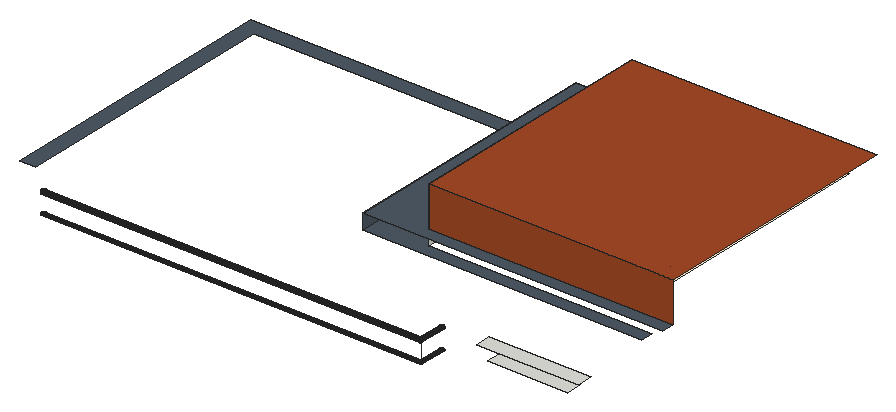
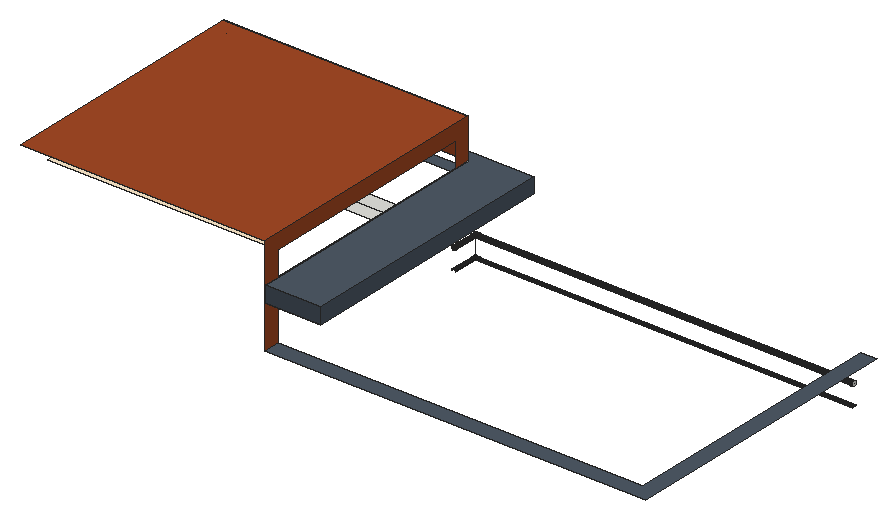
# SketchUp Ruby script. Lengths in inches.
U = 1.inch
M = Sketchup.active_model
def pt(a) = Geom::Point3d.new(a.map { |v| v * U })
def face(e, loops, mat)
  f = e.add_face(loops[0].map { |a| pt(a) })
  loops[1..].each { |l| e.add_face(l.map { |a| pt(a) }).erase! }
  f.material = f.back_material = mat if mat
  f
end
# faces: each face lists its corners as indices into pts; further lists are holes
def faces(e, pts, list, mat = nil) = list.each { |f| face(e, (f[0].is_a?(Array) ? f : [f]).map { |l| l.map { |i| pts[i] } }, mat) }
# xy, xz, yz: faces in a plane at the given z, y or x. An outline is a flat list of corners, or four numbers for a rectangle; further outlines are holes
def ring(l) = l.size == 4 ? [[l[0], l[1]], [l[2], l[1]], [l[2], l[3]], [l[0], l[3]]] : l.each_slice(2).to_a
def flat(e, list, mat, &to3) = list.each { |f| face(e, (f[0].is_a?(Array) ? f : [f]).map { |l| ring(l).map { |u, v| to3.(u, v) } }, mat) }
def xy(e, z, list, mat = nil) = flat(e, list, mat) { |x, y| [x, y, z] }
def xz(e, y, list, mat = nil) = flat(e, list, mat) { |x, z| [x, y, z] }
def yz(e, x, list, mat = nil) = flat(e, list, mat) { |y, z| [x, y, z] }
def lines(e, pts, list) = list.each { |a, b| e.add_line(pt(pts[a]), pt(pts[b])) }
# prism: a flat outline (further loops are holes) pulled along v
def prism(e, loops, v, mat = nil)
  f = face(e, loops, mat); d = Geom::Vector3d.new(v.map { |x| x * U })
  f.pushpull(f.normal.samedirection?(d) ? d.length : -d.length)
end
def box(e, o, s, mat = nil) = prism(e, [[o, [o[0] + s[0], o[1], o[2]], [o[0] + s[0], o[1] + s[1], o[2]], [o[0], o[1] + s[1], o[2]]]], [0, 0, s[2]], mat)
def at(x, y, z, deg = 0) = Geom::Transformation.translation(pt([x, y, z])) * Geom::Transformation.rotation(ORIGIN, Z_AXIS, deg.degrees)
def axes(o, x, y, z) = Geom::Transformation.new([*x, 0, *y, 0, *z, 0, *pt(o).to_a, 1])
def part(name) = M.definitions.add(name)
# library, detail: a bought-in or finely detailed component or shape, given as its bounding box
def library(name, o, s) = part(name).tap { |d| box(d.entities, o, s) }
def detail(e, o, s) = box(e.add_group.entities, o, s)
def put(e, d, t, mat = nil) = e.add_instance(d, t).tap { |i| i.material = mat if mat }
def group(e, t, mat = nil) = e.add_group.tap { |g| g.transformation = t; g.material = mat if mat }.entities
root = M.entities
M.materials.add("[0029_BlanchedAlmond]").color = [255, 235, 205]
M.materials.add("[0047_Khaki]").color = [240, 230, 140]
M.materials.add("[0111_SlateGray]").color = [79, 90, 102]
M.materials.add("[0136_Charcoal]").color = [35, 35, 35]
M.materials.add("[Cladding Siding Tan]").color = [162, 73, 37]
xy(root,2520,[[2669.375,1132.62,2981.375,1192.62]])
xy(root,2536.5,[[2448.125,1082.62,2448.96,1082.66,2449.79,1082.79,2450.6,1083.01,2451.38,1083.31,2452.125,1083.6875,2452.83,1084.15,2453.48,1084.67,2454.07,1085.26,2454.6,1085.92,2455.05,1086.62,2455.43,1087.36,2455.73,1088.15,2455.95,1088.95,2456.08,1089.78,2456.125,1090.62,2456.08,1091.45,2455.95,1092.28,2455.73,1093.09,2455.43,1093.87,2455.05,1094.62,2454.6,1095.32,2454.07,1095.97,2453.48,1096.5625,2452.83,1097.09,2452.125,1097.55,2451.38,1097.93,2450.6,1098.23,2449.79,1098.44,2448.96,1098.57,2448.125,1098.62,2447.29,1098.57,2446.46,1098.44,2445.65,1098.23,2444.87,1097.93,2444.125,1097.55,2443.42,1097.09,2442.77,1096.5625,2442.18,1095.97,2441.65,1095.32,2441.19,1094.62,2440.81,1093.87,2440.51,1093.09,2440.3,1092.28,2440.17,1091.45,2440.125,1090.62,2440.17,1089.78,2440.3,1088.95,2440.51,1088.15,2440.81,1087.36,2441.19,1086.62,2441.65,1085.92,2442.18,1085.26,2442.77,1084.67,2443.42,1084.15,2444.125,1083.6875,2444.87,1083.31,2445.65,1083.01,2446.46,1082.79,2447.29,1082.66]])
xy(root,2562,[[2627.375,1132.62,3023.375,1192.62]])
xy(root,2630.25,[[917.375,1060.62,977.375,1060.62,977.375,2116.62,2393.375,2116.62,2393.375,2176.62,917.375,2176.62]],"[0111_SlateGray]")
xy(root,2796,[[2275.57,1241.83,2272.48,1242.38,2269.65,1243.71,2267.25,1245.73,2265.46,1248.3,2264.4,1251.25,2264.13,1254.37,2264.68,1257.46,2266.01,1260.29,2268.03,1262.6875,2270.6,1264.48,2273.55,1265.54,2276.67,1265.81,2279.75,1265.26,2282.59,1263.93,2284.98,1261.91,2286.77,1259.34,2287.84,1256.39,2288.11,1253.27,2287.55,1250.19,2286.22,1247.35,2284.2,1244.95,2281.63,1243.16,2278.6875,1242.1],[2275.57,1421.83,2272.48,1422.38,2269.65,1423.71,2267.25,1425.73,2265.46,1428.3,2264.4,1431.25,2264.13,1434.37,2264.68,1437.46,2266.01,1440.29,2268.03,1442.6875,2270.6,1444.48,2273.55,1445.54,2276.67,1445.81,2279.75,1445.26,2282.59,1443.93,2284.98,1441.91,2286.77,1439.34,2287.84,1436.39,2288.11,1433.27,2287.55,1430.19,2286.22,1427.35,2284.2,1424.95,2281.63,1423.16,2278.6875,1422.1],[2275.57,1601.83,2272.48,1602.38,2269.65,1603.71,2267.25,1605.73,2265.46,1608.3,2264.4,1611.25,2264.13,1614.37,2264.68,1617.46,2266.01,1620.29,2268.03,1622.6875,2270.6,1624.48,2273.55,1625.54,2276.67,1625.81,2279.75,1625.26,2282.59,1623.93,2284.98,1621.91,2286.77,1619.34,2287.84,1616.39,2288.11,1613.27,2287.55,1610.19,2286.22,1607.35,2284.2,1604.95,2281.63,1603.16,2278.6875,1602.1],[2275.57,1781.83,2272.48,1782.38,2269.65,1783.71,2267.25,1785.73,2265.46,1788.3,2264.4,1791.25,2264.13,1794.37,2264.68,1797.46,2266.01,1800.29,2268.03,1802.6875,2270.6,1804.48,2273.55,1805.54,2276.67,1805.81,2279.75,1805.26,2282.59,1803.93,2284.98,1801.91,2286.77,1799.34,2287.84,1796.39,2288.11,1793.27,2287.55,1790.19,2286.22,1787.35,2284.2,1784.95,2281.63,1783.16,2278.6875,1782.1],[2275.57,1961.83,2272.48,1962.38,2269.65,1963.71,2267.25,1965.73,2265.46,1968.3,2264.4,1971.25,2264.13,1974.37,2264.68,1977.46,2266.01,1980.29,2268.03,1982.6875,2270.6,1984.48,2273.55,1985.54,2276.67,1985.81,2279.75,1985.26,2282.59,1983.93,2284.98,1981.91,2286.77,1979.34,2287.84,1976.39,2288.11,1973.27,2287.55,1970.19,2286.22,1967.35,2284.2,1964.95,2281.63,1963.16,2278.6875,1962.1]],"[0047_Khaki]")
xy(root,2796,[[[2177.375,1144.62,2177.375,2176.62,2393.375,2176.62,2393.375,1192.62,3257.375,1192.62,3257.375,1144.62],[2275.57,1421.83,2278.6875,1422.1,2281.63,1423.16,2284.2,1424.95,2286.22,1427.35,2287.55,1430.19,2288.11,1433.27,2287.84,1436.39,2286.77,1439.34,2284.98,1441.91,2282.59,1443.93,2279.75,1445.26,2276.67,1445.81,2273.55,1445.54,2270.6,1444.48,2268.03,1442.6875,2266.01,1440.29,2264.68,1437.46,2264.13,1434.37,2264.4,1431.25,2265.46,1428.3,2267.25,1425.73,2269.65,1423.71,2272.48,1422.38],[2275.57,1781.83,2278.6875,1782.1,2281.63,1783.16,2284.2,1784.95,2286.22,1787.35,2287.55,1790.19,2288.11,1793.27,2287.84,1796.39,2286.77,1799.34,2284.98,1801.91,2282.59,1803.93,2279.75,1805.26,2276.67,1805.81,2273.55,1805.54,2270.6,1804.48,2268.03,1802.6875,2266.01,1800.29,2264.68,1797.46,2264.13,1794.37,2264.4,1791.25,2265.46,1788.3,2267.25,1785.73,2269.65,1783.71,2272.48,1782.38],[2275.57,1601.83,2278.6875,1602.1,2281.63,1603.16,2284.2,1604.95,2286.22,1607.35,2287.55,1610.19,2288.11,1613.27,2287.84,1616.39,2286.77,1619.34,2284.98,1621.91,2282.59,1623.93,2279.75,1625.26,2276.67,1625.81,2273.55,1625.54,2270.6,1624.48,2268.03,1622.6875,2266.01,1620.29,2264.68,1617.46,2264.13,1614.37,2264.4,1611.25,2265.46,1608.3,2267.25,1605.73,2269.65,1603.71,2272.48,1602.38],[2275.57,1961.83,2278.6875,1962.1,2281.63,1963.16,2284.2,1964.95,2286.22,1967.35,2287.55,1970.19,2288.11,1973.27,2287.84,1976.39,2286.77,1979.34,2284.98,1981.91,2282.59,1983.93,2279.75,1985.26,2276.67,1985.81,2273.55,1985.54,2270.6,1984.48,2268.03,1982.6875,2266.01,1980.29,2264.68,1977.46,2264.13,1974.37,2264.4,1971.25,2265.46,1968.3,2267.25,1965.73,2269.65,1963.71,2272.48,1962.38],[2275.57,1241.83,2278.6875,1242.1,2281.63,1243.16,2284.2,1244.95,2286.22,1247.35,2287.55,1250.19,2288.11,1253.27,2287.84,1256.39,2286.77,1259.34,2284.98,1261.91,2282.59,1263.93,2279.75,1265.26,2276.67,1265.81,2273.55,1265.54,2270.6,1264.48,2268.03,1262.6875,2266.01,1260.29,2264.68,1257.46,2264.13,1254.37,2264.4,1251.25,2265.46,1248.3,2267.25,1245.73,2269.65,1243.71,2272.48,1242.38]]],"[0111_SlateGray]")
xy(root,2856,[[2177.375,1144.62,3341.375,1144.62,3341.375,1192.62,2393.375,1192.62,2393.375,2176.62,2177.375,2176.62]],"[0111_SlateGray]")
xy(root,2952,[[2393.375,1252.62,3281.375,2116.62]],"[0029_BlanchedAlmond]")
xy(root,3012,[[2393.375,1192.62,3341.375,2176.62]],"[Cladding Siding Tan]")
xz(root,1192.62,[[2393.375,2856,3341.375,3012]],"[Cladding Siding Tan]")
xz(root,2176.62,[[2177.375,2796,2393.375,2856]],"[0111_SlateGray]")
yz(root,977.375,[[1090.62,2527,1089.78,2527.04,1088.95,2527.17,1088.15,2527.39,1087.36,2527.69,1086.62,2528.07,1085.92,2528.53,1085.26,2529.05,1084.67,2529.65,1084.15,2530.3,1083.6875,2531,1083.31,2531.75,1083.01,2532.53,1082.79,2533.34,1082.66,2534.16,1082.62,2535,1082.66,2535.84,1082.79,2536.66,1083.01,2537.47,1083.31,2538.25,1083.6875,2539,1084.15,2539.7,1084.67,2540.35,1085.26,2540.95,1085.92,2541.47,1086.62,2541.93,1087.36,2542.31,1088.15,2542.61,1088.95,2542.83,1089.78,2542.96,1090.62,2543,1091.45,2542.96,1092.28,2542.83,1093.09,2542.61,1093.87,2542.31,1094.62,2541.93,1095.32,2541.47,1095.97,2540.95,1096.5625,2540.35,1097.09,2539.7,1097.55,2539,1097.93,2538.25,1098.23,2537.47,1098.44,2536.66,1098.57,2535.84,1098.62,2535,1098.57,2534.16,1098.44,2533.34,1098.23,2532.53,1097.93,2531.75,1097.55,2531,1097.09,2530.3,1096.5625,2529.65,1095.97,2529.05,1095.32,2528.53,1094.62,2528.07,1093.87,2527.69,1093.09,2527.39,1092.28,2527.17,1091.45,2527.04]])
yz(root,2177.375,[[1144.62,2796,2176.62,2856]],"[0111_SlateGray]")
yz(root,2393.375,[[1192.62,2796,1252.62,2856],[1252.62,2796,2116.62,2856],[2116.62,2796,2176.62,2856]])
yz(root,2393.375,[[2116.62,2630.25,2176.62,2796],[1192.62,2856,1192.62,3012,2176.62,3012,2176.62,2856,2116.62,2856,2116.62,2952,1252.62,2952,1252.62,2856]],"[Cladding Siding Tan]")
p = [[977.375,1083.01,2456.47],[977.375,1082.79,2455.66],[2446.46,1082.79,2455.66],[2449.79,1082.79,2455.66],[2455.95,1082.79,2455.66],[2455.73,1083.01,2456.47],
  [2450.6,1083.01,2456.47],[2445.65,1083.01,2456.47],[2455.95,1088.95,2455.66],[2455.95,1092.28,2455.66],[2455.95,1192.62,2455.66],[2455.73,1192.62,2456.47],
  [2455.73,1093.09,2456.47],[2455.73,1088.15,2456.47],[977.375,1098.44,2455.66],[977.375,1098.23,2456.47],[2440.51,1098.23,2456.47],[2440.3,1098.44,2455.66],
  [2440.51,1192.62,2456.47],[2440.3,1192.62,2455.66],[977.375,1083.31,2457.25],[2455.43,1083.31,2457.25],[2451.38,1083.31,2457.25],[2444.87,1083.31,2457.25],
  [2455.43,1192.62,2457.25],[2455.43,1093.87,2457.25],[2455.43,1087.36,2457.25],[977.375,1097.93,2457.25],[2440.81,1097.93,2457.25],[2440.81,1192.62,2457.25],
  [977.375,1083.6875,2458],[2455.05,1083.6875,2458],[2452.125,1083.6875,2458],[2444.125,1083.6875,2458],[2455.05,1192.62,2458],[2455.05,1094.62,2458],
  [2455.05,1086.62,2458],[977.375,1097.55,2458],[2441.19,1097.55,2458],[2441.19,1192.62,2458],[977.375,1084.15,2458.7],[2454.6,1084.15,2458.7],
  [2452.83,1084.15,2458.7],[2443.42,1084.15,2458.7],[2454.6,1192.62,2458.7],[2454.6,1095.32,2458.7],[2454.6,1085.92,2458.7],[977.375,1097.09,2458.7],
  [2441.65,1097.09,2458.7],[2441.65,1192.62,2458.7],[977.375,1084.67,2459.35],[2454.07,1084.67,2459.35],[2453.48,1084.67,2459.35],[2442.77,1084.67,2459.35],
  [2454.07,1192.62,2459.35],[2454.07,1095.97,2459.35],[2454.07,1085.26,2459.35],[977.375,1096.5625,2459.35],[2442.18,1096.5625,2459.35],[2442.18,1192.62,2459.35],
  [977.375,1085.26,2459.95],[2453.48,1085.26,2459.95],[2442.18,1085.26,2459.95],[2453.48,1192.62,2459.95],[2453.48,1096.5625,2459.95],[977.375,1095.97,2459.95],
  [2442.18,1095.97,2459.95],[2442.77,1095.97,2459.95],[2442.77,1096.5625,2459.95],[2442.77,1192.62,2459.95],[977.375,1085.92,2460.47],[2452.83,1085.92,2460.47],
  [2441.65,1085.92,2460.47],[2452.83,1192.62,2460.47],[2452.83,1097.09,2460.47],[977.375,1095.32,2460.47],[2441.65,1095.32,2460.47],[2443.42,1095.32,2460.47],
  [2443.42,1097.09,2460.47],[2443.42,1192.62,2460.47],[977.375,1086.62,2460.93],[2452.125,1086.62,2460.93],[2441.19,1086.62,2460.93],[2452.125,1192.62,2460.93],
  [2452.125,1097.55,2460.93],[977.375,1094.62,2460.93],[2441.19,1094.62,2460.93],[2444.125,1094.62,2460.93],[2444.125,1097.55,2460.93],[2444.125,1192.62,2460.93],
  [977.375,1087.36,2461.31],[2451.38,1087.36,2461.31],[2440.81,1087.36,2461.31],[2451.38,1192.62,2461.31],[2451.38,1097.93,2461.31],[977.375,1093.87,2461.31],
  [2440.81,1093.87,2461.31],[2444.87,1093.87,2461.31],[2444.87,1097.93,2461.31],[2444.87,1192.62,2461.31],[977.375,1088.15,2461.61],[2450.6,1088.15,2461.61],
  [2440.51,1088.15,2461.61],[2450.6,1192.62,2461.61],[2450.6,1098.23,2461.61],[977.375,1093.09,2461.61],[2440.51,1093.09,2461.61],[2445.65,1093.09,2461.61],
  [2445.65,1098.23,2461.61],[2445.65,1192.62,2461.61],[977.375,1088.95,2461.83],[2449.79,1088.95,2461.83],[2440.3,1088.95,2461.83],[2449.79,1192.62,2461.83],
  [2449.79,1098.44,2461.83],[977.375,1092.28,2461.83],[2440.3,1092.28,2461.83],[2446.46,1092.28,2461.83],[2446.46,1098.44,2461.83],[2446.46,1192.62,2461.83],
  [977.375,1089.78,2461.96],[2448.96,1089.78,2461.96],[2440.17,1089.78,2461.96],[2448.96,1192.62,2461.96],[2448.96,1098.57,2461.96],[977.375,1091.45,2461.96],
  [2440.17,1091.45,2461.96],[2447.29,1091.45,2461.96],[2447.29,1098.57,2461.96],[2447.29,1192.62,2461.96],[977.375,1090.62,2462],[2448.125,1090.62,2462],
  [2440.125,1090.62,2462],[2448.125,1192.62,2462],[2448.125,1098.62,2462],[977.375,1088.95,2527.17],[977.375,1089.78,2527.04],[2440.17,1089.78,2527.04],
  [2448.96,1089.78,2527.04],[2449.79,1088.95,2527.17],[2440.3,1088.95,2527.17],[2448.96,1098.57,2527.04],[2448.96,1192.62,2527.04],[2449.79,1192.62,2527.17],
  [2449.79,1098.44,2527.17],[977.375,1090.62,2527],[2440.125,1090.62,2527],[2448.125,1090.62,2527],[2448.125,1098.62,2527],[2448.125,1192.62,2527],
  [977.375,1091.45,2527.04],[2440.17,1091.45,2527.04],[2447.29,1091.45,2527.04],[2447.29,1098.57,2527.04],[2447.29,1192.62,2527.04],[977.375,1092.28,2527.17],
  [2440.3,1092.28,2527.17],[2446.46,1092.28,2527.17],[2446.46,1098.44,2527.17],[2446.46,1192.62,2527.17],[977.375,1088.15,2527.39],[2450.6,1088.15,2527.39],
  [2440.51,1088.15,2527.39],[2450.6,1192.62,2527.39],[2450.6,1098.23,2527.39],[977.375,1093.09,2527.39],[2440.51,1093.09,2527.39],[2445.65,1093.09,2527.39],
  [2445.65,1098.23,2527.39],[2445.65,1192.62,2527.39],[977.375,1087.36,2527.69],[2451.38,1087.36,2527.69],[2440.81,1087.36,2527.69],[2451.38,1192.62,2527.69],
  [2451.38,1097.93,2527.69],[977.375,1093.87,2527.69],[2440.81,1093.87,2527.69],[2444.87,1093.87,2527.69],[2444.87,1097.93,2527.69],[2444.87,1192.62,2527.69],
  [977.375,1086.62,2528.07],[2452.125,1086.62,2528.07],[2441.19,1086.62,2528.07],[2452.125,1192.62,2528.07],[2452.125,1097.55,2528.07],[977.375,1094.62,2528.07],
  [2441.19,1094.62,2528.07],[2444.125,1094.62,2528.07],[2444.125,1097.55,2528.07],[2444.125,1192.62,2528.07],[977.375,1085.92,2528.53],[2452.83,1085.92,2528.53],
  [2441.65,1085.92,2528.53],[2452.83,1192.62,2528.53],[2452.83,1097.09,2528.53],[977.375,1095.32,2528.53],[2441.65,1095.32,2528.53],[2443.42,1095.32,2528.53],
  [2443.42,1097.09,2528.53],[2443.42,1192.62,2528.53],[977.375,1085.26,2529.05],[2453.48,1085.26,2529.05],[2442.18,1085.26,2529.05],[2453.48,1192.62,2529.05],
  [2453.48,1096.5625,2529.05],[977.375,1095.97,2529.05],[2442.18,1095.97,2529.05],[2442.77,1095.97,2529.05],[2442.77,1096.5625,2529.05],[2442.77,1192.62,2529.05],
  [977.375,1084.67,2529.65],[2454.07,1084.67,2529.65],[2453.48,1084.67,2529.65],[2442.77,1084.67,2529.65],[2454.07,1192.62,2529.65],[2454.07,1095.97,2529.65],
  [2454.07,1085.26,2529.65],[977.375,1096.5625,2529.65],[2442.18,1096.5625,2529.65],[2442.18,1192.62,2529.65],[977.375,1084.15,2530.3],[2454.6,1084.15,2530.3],
  [2452.83,1084.15,2530.3],[2443.42,1084.15,2530.3],[2454.6,1192.62,2530.3],[2454.6,1095.32,2530.3],[2454.6,1085.92,2530.3],[977.375,1097.09,2530.3],
  [2441.65,1097.09,2530.3],[2441.65,1192.62,2530.3],[977.375,1083.6875,2531],[2455.05,1083.6875,2531],[2452.125,1083.6875,2531],[2444.125,1083.6875,2531],
  [2455.05,1192.62,2531],[2455.05,1094.62,2531],[2455.05,1086.62,2531],[977.375,1097.55,2531],[2441.19,1097.55,2531],[2441.19,1192.62,2531],
  [977.375,1083.31,2531.75],[2455.43,1083.31,2531.75],[2451.38,1083.31,2531.75],[2444.87,1083.31,2531.75],[2455.43,1192.62,2531.75],[2455.43,1093.87,2531.75],
  [2455.43,1087.36,2531.75],[977.375,1097.93,2531.75],[2440.81,1097.93,2531.75],[2440.81,1192.62,2531.75],[977.375,1083.01,2532.53],[2455.73,1083.01,2532.53],
  [2450.6,1083.01,2532.53],[2445.65,1083.01,2532.53],[2455.73,1192.62,2532.53],[2455.73,1093.09,2532.53],[2455.73,1088.15,2532.53],[977.375,1098.23,2532.53],
  [2440.51,1098.23,2532.53],[2440.51,1192.62,2532.53],[977.375,1082.79,2533.34],[2455.95,1082.79,2533.34],[2449.79,1082.79,2533.34],[2446.46,1082.79,2533.34],
  [2455.95,1192.62,2533.34],[2455.95,1092.28,2533.34],[2455.95,1088.95,2533.34],[977.375,1098.44,2533.34],[2440.3,1098.44,2533.34],[2440.3,1192.62,2533.34],
  [977.375,1082.66,2534.16],[2456.08,1082.66,2534.16],[2448.96,1082.66,2534.16],[2447.29,1082.66,2534.16],[2456.08,1192.62,2534.16],[2456.08,1091.45,2534.16],
  [2456.08,1089.78,2534.16],[977.375,1098.57,2534.16],[2440.17,1098.57,2534.16],[2440.17,1192.62,2534.16],[977.375,1082.62,2535],[2456.125,1082.62,2535],
  [2448.125,1082.62,2535],[2456.125,1192.62,2535],[2456.125,1090.62,2535],[977.375,1098.62,2535],[2440.125,1098.62,2535],[2440.125,1192.62,2535],
  [977.375,1082.66,2535.84],[2456.08,1082.66,2535.84],[2448.96,1082.66,2535.84],[2447.29,1082.66,2535.84],[2456.08,1192.62,2535.84],[2456.08,1091.45,2535.84],
  [2456.08,1089.78,2535.84],[977.375,1098.57,2535.84],[2440.17,1098.57,2535.84],[2440.17,1192.62,2535.84],[977.375,1082.79,2536.66],[2455.95,1082.79,2536.66],
  [2449.79,1082.79,2536.66],[2446.46,1082.79,2536.66],[2455.95,1192.62,2536.66],[2455.95,1092.28,2536.66],[2455.95,1088.95,2536.66],[977.375,1098.44,2536.66],
  [2440.3,1098.44,2536.66],[2440.3,1192.62,2536.66],[977.375,1083.01,2537.47],[2455.73,1083.01,2537.47],[2450.6,1083.01,2537.47],[2445.65,1083.01,2537.47],
  [2455.73,1192.62,2537.47],[2455.73,1093.09,2537.47],[2455.73,1088.15,2537.47],[977.375,1098.23,2537.47],[2440.51,1098.23,2537.47],[2440.51,1192.62,2537.47],
  [977.375,1083.31,2538.25],[2455.43,1083.31,2538.25],[2451.38,1083.31,2538.25],[2444.87,1083.31,2538.25],[2455.43,1192.62,2538.25],[2455.43,1093.87,2538.25],
  [2455.43,1087.36,2538.25],[977.375,1097.93,2538.25],[2440.81,1097.93,2538.25],[2440.81,1192.62,2538.25],[977.375,1083.6875,2539],[2455.05,1083.6875,2539],
  [2452.125,1083.6875,2539],[2444.125,1083.6875,2539],[2455.05,1192.62,2539],[2455.05,1094.62,2539],[2455.05,1086.62,2539],[977.375,1097.55,2539],
  [2441.19,1097.55,2539],[2441.19,1192.62,2539],[977.375,1084.15,2539.7],[2454.6,1084.15,2539.7],[2452.83,1084.15,2539.7],[2443.42,1084.15,2539.7],
  [2454.6,1192.62,2539.7],[2454.6,1095.32,2539.7],[2454.6,1085.92,2539.7],[977.375,1097.09,2539.7],[2441.65,1097.09,2539.7],[2441.65,1192.62,2539.7],
  [977.375,1084.67,2540.35],[2454.07,1084.67,2540.35],[2453.48,1084.67,2540.35],[2442.77,1084.67,2540.35],[2454.07,1192.62,2540.35],[2454.07,1095.97,2540.35],
  [2454.07,1085.26,2540.35],[977.375,1096.5625,2540.35],[2442.18,1096.5625,2540.35],[2442.18,1192.62,2540.35],[977.375,1085.26,2540.95],[2453.48,1085.26,2540.95],
  [2442.18,1085.26,2540.95],[2453.48,1192.62,2540.95],[2453.48,1096.5625,2540.95],[977.375,1095.97,2540.95],[2442.18,1095.97,2540.95],[2442.77,1095.97,2540.95],
  [2442.77,1096.5625,2540.95],[2442.77,1192.62,2540.95],[977.375,1085.92,2541.47],[2452.83,1085.92,2541.47],[2441.65,1085.92,2541.47],[2452.83,1192.62,2541.47],
  [2452.83,1097.09,2541.47],[977.375,1095.32,2541.47],[2441.65,1095.32,2541.47],[2443.42,1095.32,2541.47],[2443.42,1097.09,2541.47],[2443.42,1192.62,2541.47],
  [977.375,1086.62,2541.93],[2452.125,1086.62,2541.93],[2441.19,1086.62,2541.93],[2452.125,1192.62,2541.93],[2452.125,1097.55,2541.93],[977.375,1094.62,2541.93],
  [2441.19,1094.62,2541.93],[2444.125,1094.62,2541.93],[2444.125,1097.55,2541.93],[2444.125,1192.62,2541.93],[977.375,1087.36,2542.31],[2451.38,1087.36,2542.31],
  [2440.81,1087.36,2542.31],[2451.38,1192.62,2542.31],[2451.38,1097.93,2542.31],[977.375,1093.87,2542.31],[2440.81,1093.87,2542.31],[2444.87,1093.87,2542.31],
  [2444.87,1097.93,2542.31],[2444.87,1192.62,2542.31],[977.375,1088.15,2542.61],[2450.6,1088.15,2542.61],[2440.51,1088.15,2542.61],[2450.6,1192.62,2542.61],
  [2450.6,1098.23,2542.61],[977.375,1093.09,2542.61],[2440.51,1093.09,2542.61],[2445.65,1093.09,2542.61],[2445.65,1098.23,2542.61],[2445.65,1192.62,2542.61],
  [977.375,1088.95,2542.83],[2449.79,1088.95,2542.83],[2440.3,1088.95,2542.83],[2449.79,1192.62,2542.83],[2449.79,1098.44,2542.83],[977.375,1092.28,2542.83],
  [2440.3,1092.28,2542.83],[2446.46,1092.28,2542.83],[2446.46,1098.44,2542.83],[2446.46,1192.62,2542.83],[977.375,1089.78,2542.96],[2448.96,1089.78,2542.96],
  [2440.17,1089.78,2542.96],[2448.96,1192.62,2542.96],[2448.96,1098.57,2542.96],[977.375,1091.45,2542.96],[2440.17,1091.45,2542.96],[2447.29,1091.45,2542.96],
  [2447.29,1098.57,2542.96],[2447.29,1192.62,2542.96],[977.375,1090.62,2543],[2448.125,1090.62,2543],[2440.125,1090.62,2543],[2448.125,1192.62,2543],
  [2448.125,1098.62,2543],[2448.125,1090.62,2535],[2440.125,1090.62,2535],[2448.125,1192.62,2535],[2448.125,1098.62,2535],[977.375,1090.62,2535],
  [2455.05,1086.62,2536.5],[2455.43,1087.36,2536.5],[2440.125,1090.62,2536.5],[2449.79,1082.79,2536.5],[2451.38,1083.31,2536.5],[2454.07,1085.26,2536.5],
  [2455.73,1088.15,2536.5],[2455.95,1088.95,2536.5],[2440.17,1089.78,2536.5],[2450.6,1083.01,2536.5],[2452.125,1083.6875,2536.5],[2452.83,1084.15,2536.5],
  [2453.48,1084.67,2536.5],[2454.6,1085.92,2536.5],[2447.29,1098.57,2536.5],[2446.46,1098.44,2536.5],[2445.65,1098.23,2536.5],[2444.87,1097.93,2536.5],
  [2444.125,1097.55,2536.5],[2443.42,1097.09,2536.5],[2442.77,1096.5625,2536.5],[2442.18,1095.97,2536.5],[2441.65,1095.32,2536.5],[2441.19,1094.62,2536.5],
  [2440.81,1093.87,2536.5],[2440.51,1093.09,2536.5],[2440.3,1092.28,2536.5],[2440.17,1091.45,2536.5],[2440.3,1088.95,2536.5],[2440.51,1088.15,2536.5],
  [2440.81,1087.36,2536.5],[2441.19,1086.62,2536.5],[2441.65,1085.92,2536.5],[2442.18,1085.26,2536.5],[2442.77,1084.67,2536.5],[2443.42,1084.15,2536.5],
  [2444.125,1083.6875,2536.5],[2444.87,1083.31,2536.5],[2445.65,1083.01,2536.5],[2446.46,1082.79,2536.5],[2455.95,1092.28,2536.5],[2455.73,1093.09,2536.5],
  [2455.43,1093.87,2536.5],[2455.05,1094.62,2536.5],[2454.6,1095.32,2536.5],[2454.07,1095.97,2536.5],[2453.48,1096.5625,2536.5],[2452.83,1097.09,2536.5],
  [2452.125,1097.55,2536.5],[2451.38,1097.93,2536.5],[2450.6,1098.23,2536.5],[2449.79,1098.44,2536.5],[2448.96,1098.57,2536.5],[2448.125,1098.62,2536.5],
  [3281.375,1252.62,2952],[3281.375,1252.62,3012]]
faces(root,p,[[0,1,2,3,4,5,6,7],[5,4,8,9,10,11,12,13],[14,15,16,17],[17,16,18,19],[20,0,7,6,5,21,22,23],[21,5,13,12,11,24,25,26],[15,27,28,16],[16,28,29,18],
  [30,20,23,22,21,31,32,33],[31,21,26,25,24,34,35,36],[27,37,38,28],[28,38,39,29],[40,30,33,32,31,41,42,43],[41,31,36,35,34,44,45,46],[37,47,48,38],[38,48,49,39],
  [50,40,43,42,41,51,52,53],[51,41,46,45,44,54,55,56],[47,57,58,48],[48,58,59,49],[60,50,53,52,51,61,62],[61,51,56,55,54,63,64],[57,65,66,67,58],[58,67,68,69,59],
  [70,60,62,61,71,72],[71,61,64,63,73,74],[65,75,76,77,67,66],[67,77,78,79,69,68],[80,70,72,71,81,82],[81,71,74,73,83,84],[75,85,86,87,77,76],[77,87,88,89,79,78],
  [90,80,82,81,91,92],[91,81,84,83,93,94],[85,95,96,97,87,86],[87,97,98,99,89,88],[100,90,92,91,101,102],[101,91,94,93,103,104],[95,105,106,107,97,96],[97,107,108,109,99,98],
  [110,100,102,101,111,112],[111,101,104,103,113,114],[105,115,116,117,107,106],[107,117,118,119,109,108],[120,110,112,111,121,122],[121,111,114,113,123,124],[115,125,126,127,117,116],[117,127,128,129,119,118],
  [130,120,122,121,131,132],[131,121,124,123,133,134],[125,130,132,131,127,126],[127,131,134,133,129,128],[135,136,137,138,139,140],[139,138,141,142,143,144],[136,145,146,147,138,137],[138,147,148,149,142,141],
  [145,150,151,152,147,146],[147,152,153,154,149,148],[150,155,156,157,152,151],[152,157,158,159,154,153],[160,135,140,139,161,162],[161,139,144,143,163,164],[155,165,166,167,157,156],[157,167,168,169,159,158],
  [170,160,162,161,171,172],[171,161,164,163,173,174],[165,175,176,177,167,166],[167,177,178,179,169,168],[180,170,172,171,181,182],[181,171,174,173,183,184],[175,185,186,187,177,176],[177,187,188,189,179,178],
  [190,180,182,181,191,192],[191,181,184,183,193,194],[185,195,196,197,187,186],[187,197,198,199,189,188],[200,190,192,191,201,202],[201,191,194,193,203,204],[195,205,206,207,197,196],[197,207,208,209,199,198],
  [210,200,202,201,211,212,213],[211,201,204,203,214,215,216],[205,217,218,207,206],[207,218,219,209,208],[220,210,213,212,211,221,222,223],[221,211,216,215,214,224,225,226],[217,227,228,218],[218,228,229,219],
  [230,220,223,222,221,231,232,233],[231,221,226,225,224,234,235,236],[227,237,238,228],[228,238,239,229],[240,230,233,232,231,241,242,243],[241,231,236,235,234,244,245,246],[237,247,248,238],[238,248,249,239],
  [250,240,243,242,241,251,252,253],[251,241,246,245,244,254,255,256],[247,257,258,248],[248,258,259,249],[260,250,253,252,251,261,262,263],[261,251,256,255,254,264,265,266],[257,267,268,258],[258,268,269,259],
  [270,260,263,262,261,271,272,273],[271,261,266,265,264,274,275,276],[267,277,278,268],[268,278,279,269],[280,270,273,272,271,281,282],[281,271,276,275,274,283,284],[277,285,286,278],[278,286,287,279],
  [288,280,282,281,289,290,291],[289,281,284,283,292,293,294],[285,295,296,286],[286,296,297,287],[298,288,291,290,289,299,300,301],[299,289,294,293,292,302,303,304],[295,305,306,296],[296,306,307,297],
  [308,298,301,300,299,309,310,311],[309,299,304,303,302,312,313,314],[305,315,316,306],[306,316,317,307],[318,308,311,310,309,319,320,321],[319,309,314,313,312,322,323,324],[315,325,326,316],[316,326,327,317],
  [328,318,321,320,319,329,330,331],[329,319,324,323,322,332,333,334],[325,335,336,326],[326,336,337,327],[338,328,331,330,329,339,340,341],[339,329,334,333,332,342,343,344],[335,345,346,336],[336,346,347,337],
  [348,338,341,340,339,349,350,351],[349,339,344,343,342,352,353,354],[345,355,356,346],[346,356,357,347],[358,348,351,350,349,359,360],[359,349,354,353,352,361,362],[355,363,364,365,356],[356,365,366,367,357],
  [368,358,360,359,369,370],[369,359,362,361,371,372],[363,373,374,375,365,364],[365,375,376,377,367,366],[378,368,370,369,379,380],[379,369,372,371,381,382],[373,383,384,385,375,374],[375,385,386,387,377,376],
  [388,378,380,379,389,390],[389,379,382,381,391,392],[383,393,394,395,385,384],[385,395,396,397,387,386],[398,388,390,389,399,400],[399,389,392,391,401,402],[393,403,404,405,395,394],[395,405,406,407,397,396],
  [408,398,400,399,409,410],[409,399,402,401,411,412],[403,413,414,415,405,404],[405,415,416,417,407,406],[418,408,410,409,419,420],[419,409,412,411,421,422],[413,423,424,425,415,414],[415,425,426,427,417,416],
  [428,418,420,419,429,430],[429,419,422,421,431,432],[423,428,430,429,425,424],[425,429,432,431,427,426]],"[0136_Charcoal]")
lines(root,p,[[433,429],[433,434],[435,149],[433,436],[147,433],[431,435],[131,147],[434,437],[436,435],[334,438],[324,439],[430,440],
  [300,441],[320,442],[354,443],[314,444],[304,445],[420,446],[310,447],[330,448],[340,449],[350,450],[344,451],[426,452],
  [416,453],[406,454],[396,455],[386,456],[376,457],[366,458],[364,459],[374,460],[384,461],[394,462],[404,463],[414,464],
  [424,465],[410,466],[400,467],[390,468],[380,469],[370,470],[360,471],[351,472],[341,473],[331,474],[321,475],[311,476],
  [301,477],[303,478],[313,479],[323,480],[333,481],[343,482],[353,483],[362,484],[372,485],[382,486],[392,487],[402,488],
  [412,489],[422,490],[432,491],[492,493]])
